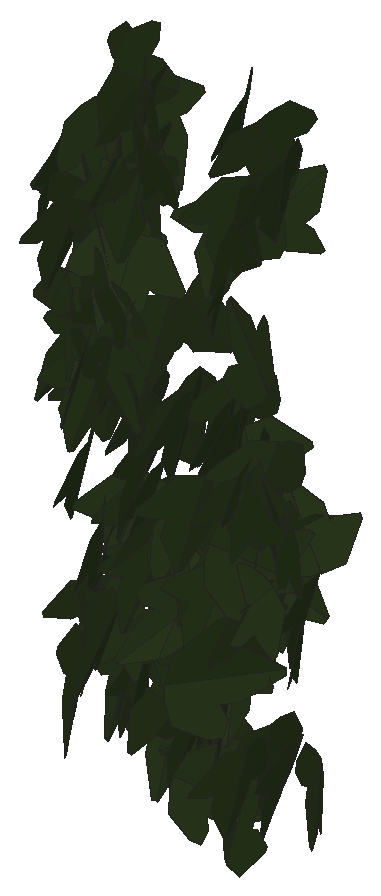
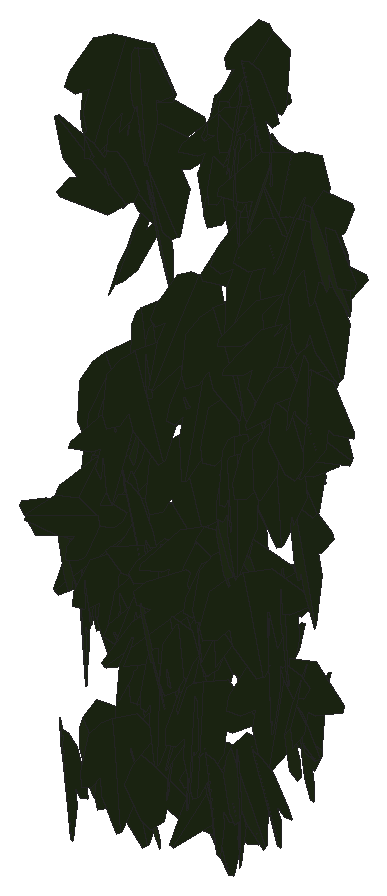
# SketchUp Ruby script. Lengths in inches.
U = 1.inch
M = Sketchup.active_model
def pt(a) = Geom::Point3d.new(a.map { |v| v * U })
def face(e, loops, mat)
  f = e.add_face(loops[0].map { |a| pt(a) })
  loops[1..].each { |l| e.add_face(l.map { |a| pt(a) }).erase! }
  f.material = f.back_material = mat if mat
  f
end
# faces: each face lists its corners as indices into pts; further lists are holes
def faces(e, pts, list, mat = nil) = list.each { |f| face(e, (f[0].is_a?(Array) ? f : [f]).map { |l| l.map { |i| pts[i] } }, mat) }
# xy, xz, yz: faces in a plane at the given z, y or x. An outline is a flat list of corners, or four numbers for a rectangle; further outlines are holes
def ring(l) = l.size == 4 ? [[l[0], l[1]], [l[2], l[1]], [l[2], l[3]], [l[0], l[3]]] : l.each_slice(2).to_a
def flat(e, list, mat, &to3) = list.each { |f| face(e, (f[0].is_a?(Array) ? f : [f]).map { |l| ring(l).map { |u, v| to3.(u, v) } }, mat) }
def xy(e, z, list, mat = nil) = flat(e, list, mat) { |x, y| [x, y, z] }
def xz(e, y, list, mat = nil) = flat(e, list, mat) { |x, z| [x, y, z] }
def yz(e, x, list, mat = nil) = flat(e, list, mat) { |y, z| [x, y, z] }
def lines(e, pts, list) = list.each { |a, b| e.add_line(pt(pts[a]), pt(pts[b])) }
# prism: a flat outline (further loops are holes) pulled along v
def prism(e, loops, v, mat = nil)
  f = face(e, loops, mat); d = Geom::Vector3d.new(v.map { |x| x * U })
  f.pushpull(f.normal.samedirection?(d) ? d.length : -d.length)
end
def box(e, o, s, mat = nil) = prism(e, [[o, [o[0] + s[0], o[1], o[2]], [o[0] + s[0], o[1] + s[1], o[2]], [o[0], o[1] + s[1], o[2]]]], [0, 0, s[2]], mat)
def at(x, y, z, deg = 0) = Geom::Transformation.translation(pt([x, y, z])) * Geom::Transformation.rotation(ORIGIN, Z_AXIS, deg.degrees)
def axes(o, x, y, z) = Geom::Transformation.new([*x, 0, *y, 0, *z, 0, *pt(o).to_a, 1])
def part(name) = M.definitions.add(name)
# library, detail: a bought-in or finely detailed component or shape, given as its bounding box
def library(name, o, s) = part(name).tap { |d| box(d.entities, o, s) }
def detail(e, o, s) = box(e.add_group.entities, o, s)
def put(e, d, t, mat = nil) = e.add_instance(d, t).tap { |i| i.material = mat if mat }
def group(e, t, mat = nil) = e.add_group.tap { |g| g.transformation = t; g.material = mat if mat }.entities
root = M.entities
M.materials.add("efeu2").color = [43, 57, 29]
c1 = part("ivyleaf_10")
p = [[0,0.5,-0.03],[-0.0625,2.02,-0.43],[-0.19,2.01,-0.46],[-0.54,1.05,-0.29],[-0.52,0.625,-0.18],[-0.83,0.76,-0.28],
  [-1.16,0.64,-0.33],[-1.15,0.33,-0.24],[-0.77,-0.39,0.02],[-0.3,-0.51,0.16],[0.04,-0.48,0.23],[-0.02,2.01,-0.4375],
  [-0.06,2.01,-0.43],[0.04,-0.49,0.23],[0.67,-0.49,0.14],[1.38,0.36,-0.2],[1.375,0.51,-0.24],[0.81,0.65,-0.19],
  [0.62,0.59,-0.15],[0.6,1.09,-0.28],[0.5,1.23,-0.31]]
faces(c1.entities,p,[[0,1,2,3,4,5,6,7,8,9,10],[11,12,0,13,14,15,16,17,18,19,20]],"efeu2")
put(root,c1,axes([506.66,136.89,179.43],[-0.21643,0.61106,0.11079],[0.02781,-0.10366,0.66875],[0.66932,0.2019,0.00804]))
put(root,c1,axes([505.3125,136.93,178.44],[0.13543,-0.68489,-0.04451],[-0.00339,0.0447,-0.69813],[0.68632,0.13537,0.00533]))
put(root,c1,axes([504.81,136.71,182.55],[-0.5524,0.19619,0.39944],[-0.38272,0.11547,-0.58598],[-0.22709,-0.67183,0.01593]))
put(root,c1,axes([504.36,137.08,181.83],[-0.27871,-0.62264,0.16039],[0.01934,-0.18285,-0.67622],[0.64267,-0.26452,0.08991]))
put(root,c1,axes([506.47,136.64,181.91],[0.09655,-0.53787,-0.44191],[0.02466,0.44851,-0.54051],[0.69569,0.05875,0.08049]))
put(root,c1,axes([503.95,136.75,179.9375],[-0.43441,0.15384,0.56092],[-0.56008,0.07816,-0.4552],[-0.15686,-0.70515,0.07191]))
put(root,c1,axes([502.98,137.33,173.17],[0.15149,-0.37032,0.60658],[0.43847,-0.43939,-0.37776],[0.5593,0.44477,0.13185]))
put(root,c1,axes([505.91,136.34,174.26],[0.04487,0.07021,0.77625],[0.10002,0.77059,-0.07548],[-0.77297,0.10379,0.03529]))
put(root,c1,axes([506.24,136.95,178.48],[0.13482,-0.67541,-0.14371],[-0.01967,0.14261,-0.68868],[0.69025,0.13599,0.00844]))
put(root,c1,axes([506.55,137.01,175.625],[0.51797,-0.07969,-0.36521],[-0.37616,0.04577,-0.50552],[0.0987,0.59265,-0.01006]))
put(root,c1,axes([503.46,137.4375,173.97],[0.14528,-0.35829,0.54775],[0.24523,-0.49042,-0.38583],[0.60685,0.28396,0.02478]))
put(root,c1,axes([504.13,137.08,180.47],[0.63313,0.2487,-0.1297],[-0.14202,0.00812,-0.67771],[-0.24187,0.64623,0.05843]))
put(root,c1,axes([503.55,137.05,178.72],[-0.56265,0.15192,-0.34681],[0.32056,-0.13943,-0.58114],[-0.20149,-0.64607,0.04387]))
put(root,c1,axes([503.22,137.18,178.59],[0.39732,-0.54573,0.04905],[0.02266,-0.04417,-0.675],[0.54746,0.3979,-0.00766]))
put(root,c1,axes([506.6,137.27,177.81],[-0.23091,-0.6062,0.20907],[0.01135,-0.22605,-0.64287],[0.64114,-0.21432,0.08668]))
put(root,c1,axes([505.92,137.08,178.4],[0.16394,-0.6525,-0.11936],[-0.00844,0.12089,-0.67245],[0.66327,0.16282,0.02095]))
put(root,c1,axes([506.42,137.01,177.4375],[-0.29178,-0.59657,-0.15254],[0.05098,0.14482,-0.66388],[0.61365,-0.29569,-0.01738]))
put(root,c1,axes([505.33,137.23,176.86],[-0.25597,-0.62666,0.1293],[-0.01982,-0.13143,-0.67622],[0.63955,-0.25488,0.03079]))
put(root,c1,axes([503.45,137.03,181.2],[-0.69675,-0.05569,0.03148],[-0.03158,-0.00006,-0.69896],[0.05563,-0.69746,-0.00245]))
put(root,c1,axes([504.34,137.17,183.06],[0.02732,-0.69814,-0.03875],[0.00552,0.039,-0.69864],[0.6992,0.02697,0.00703]))
put(root,c1,axes([506.05,137.34,181.61],[-0.46263,-0.44426,0.27239],[-0.09232,-0.2886,-0.62751],[0.51287,-0.45269,0.13274]))
put(root,c1,axes([506.11,137.22,172.65],[-0.06613,-0.65872,0.04144],[0.00583,-0.04223,-0.66195],[0.65999,-0.06563,0.01]))
put(root,c1,axes([506.07,137.29,182.04],[-0.1986,-0.65229,0.13406],[0.03584,-0.15016,-0.67754],[0.66495,-0.18672,0.07656]))
put(root,c1,axes([506.64,136.89,177.4],[0.06855,-0.55851,-0.40083],[0.15609,0.40495,-0.53754],[0.6695,-0.03722,0.16637]))
put(root,c1,axes([503.87,137.39,179],[0.10163,-0.64984,0.18183],[0.03825,-0.17804,-0.65766],[0.67371,0.10813,0.00991]))
put(root,c1,axes([504.1,137.14,182.08],[0.0796,-0.68003,-0.18076],[-0.01267,0.1805,-0.68462],[0.70353,0.08019,0.00812]))
put(root,c1,axes([503.42,137.125,181.47],[-0.35345,0.60457,-0.05381],[0.01586,-0.05305,-0.70019],[-0.60676,-0.35356,0.01305]))
put(root,c1,axes([504.27,136.8,183.66],[-0.04668,-0.43629,-0.5854],[0.18974,0.55919,-0.43189],[0.70502,-0.17938,0.07747]))
put(root,c1,axes([503.72,137.11,179.66],[-0.64262,0.23144,0.02187],[-0.02769,-0.01237,-0.6827],[-0.23081,-0.64287,0.02101]))
put(root,c1,axes([504.39,137.2,182.12],[-0.03664,-0.68496,-0.10572],[0.03027,0.10418,-0.6855],[0.6924,-0.0408,0.02437]))
put(root,c1,axes([502.67,137.4,181.62],[0.28007,-0.6353,0.11245],[0.03092,-0.10923,-0.69412],[0.64443,0.28134,-0.01556]))
put(root,c1,axes([505.82,137.27,180.87],[0.34369,-0.60969,-0.07957],[-0.01815,0.08106,-0.69948],[0.61459,0.34334,0.02384]))
put(root,c1,axes([505.13,137.5,173.1],[0.07976,-0.62324,0.17864],[0.00084,-0.17988,-0.62797],[0.64834,0.07691,-0.02116]))
put(root,c1,axes([503.51,137.34,181.25],[0.69596,-0.00157,-0.05339],[-0.05322,0.03876,-0.69489],[0.00453,0.69693,0.03853]))
put(root,c1,axes([504.35,137.33,182.99],[-0.4304,0.54258,-0.14674],[-0.00583,-0.18912,-0.68218],[-0.56204,-0.41354,0.11945]))
put(root,c1,axes([502.78,137.47,180.58],[0.01162,-0.69001,0.11879],[-0.00644,-0.11891,-0.69006],[0.70013,0.01036,-0.00832]))
put(root,c1,axes([503.91,137.43,181.92],[0.58075,-0.39263,-0.0221],[-0.02788,-0.00178,-0.70081],[0.39226,0.58117,-0.01708]))
put(root,c1,axes([506.32,137.23,177.64],[0.14089,-0.62519,-0.23745],[0.00462,0.24357,-0.63855],[0.66874,0.13003,0.05444]))
put(root,c1,axes([502.94,137.74,178.64],[-0.00213,-0.4887,0.47237],[-0.00674,-0.47234,-0.4887],[0.67965,-0.00621,-0.00337]))
put(root,c1,axes([503.21,137.59,178.09],[-0.19051,-0.60733,0.2591],[0.0341,-0.27836,-0.6274],[0.65941,-0.16107,0.10731]))
put(root,c1,axes([503.77,137.44,182.36],[-0.35837,0.49503,-0.3433],[0.20812,-0.27312,-0.61108],[-0.56532,-0.41435,-0.00735]))
put(root,c1,axes([504.45,137.52,179.38],[-0.25696,-0.62563,0.16499],[0.00234,-0.17842,-0.67292],[0.64701,-0.24782,0.06796]))
put(root,c1,axes([504.97,137.24,178.22],[-0.08665,-0.63688,-0.23448],[0.10679,0.22065,-0.63877],[0.67022,-0.1175,0.07147]))
put(root,c1,axes([504.88,137.65,174.63],[0.34102,0.2431,-0.52089],[-0.41829,-0.31049,-0.41875],[-0.39428,0.53965,-0.00628]))
put(root,c1,axes([506.3125,137.24,175.17],[-0.10941,-0.60226,-0.2658],[0.06667,0.25792,-0.61186],[0.65492,-0.12687,0.01789]))
put(root,c1,axes([505.4375,136.97,172.13],[0.06842,0.33467,0.54829],[0.08467,0.52145,-0.35406],[-0.66908,0.10021,0.01126]))
put(root,c1,axes([503.37,137.33,175.45],[0.22157,-0.58135,-0.21067],[-0.00976,0.22047,-0.61866],[0.61826,0.21182,0.06573]))
put(root,c1,axes([506.7,137.37,182.54],[0.0611,-0.67943,-0.17144],[-0.0158,0.17071,-0.68217],[0.70055,0.06311,-0.00044]))
put(root,c1,axes([504.02,137.34,183.48],[0.5103,-0.4078,-0.26684],[-0.14992,0.23627,-0.64778],[0.46371,0.52515,0.08422]))
put(root,c1,axes([505.46,137.71,173.59],[0.36769,-0.41825,0.37265],[0.27909,-0.24972,-0.55565],[0.4857,0.46011,0.03718]))
put(root,c1,axes([502.87,137.85,173.57],[0.05963,-0.17735,0.64298],[0.44796,-0.46763,-0.17053],[0.49417,0.4453,0.07699]))
put(root,c1,axes([505.51,137.66,175.19],[-0.30867,-0.51924,0.28521],[-0.10029,-0.27116,-0.6022],[0.58386,-0.32108,0.04734]))
put(root,c1,axes([506.15,136.9375,176.25],[0.00906,0.43631,0.61013],[0.01633,0.60992,-0.4364],[-0.74991,0.01856,-0.00214]))
put(root,c1,axes([506.125,137.72,175],[0.0423,0.42577,-0.44116],[-0.2339,-0.38654,-0.42429],[-0.60549,0.17906,0.13308]))
put(root,c1,axes([506.23,137.36,177.4],[-0.53939,0.42186,0.01176],[-0.00666,0.01057,-0.68476],[-0.42198,-0.53942,-0.00423]))
put(root,c1,axes([502.99,137.48,176.6],[0.21073,-0.62079,-0.12843],[-0.0454,0.12022,-0.65556],[0.6323,0.21552,-0.00427]))
put(root,c1,axes([502.98,137.7,179.27],[0.16354,0.59311,-0.30164],[-0.06851,-0.29395,-0.61515],[-0.66187,0.17698,-0.01085]))
put(root,c1,axes([504.09,137.43,182.22],[0.20776,-0.62379,-0.25004],[-0.0017,0.26123,-0.65311],[0.67204,0.1935,0.07565]))
put(root,c1,axes([504.3,137.42,177.92],[-0.57645,0.16029,0.35396],[-0.3481,0.06832,-0.59786],[-0.17264,-0.67299,0.02361]))
put(root,c1,axes([503.375,137.38,182.28],[0.32176,0.59895,0.15796],[-0.08213,0.21767,-0.6581],[-0.61396,0.28477,0.17081]))
put(root,c1,axes([504.27,137.375,182.78],[0.04732,0.67843,0.19217],[0.013,0.19173,-0.68008],[-0.705,0.04907,0.00036]))
put(root,c1,axes([505.43,137.9375,174.625],[-0.27454,-0.26666,0.55039],[-0.30057,-0.46658,-0.37599],[0.53263,-0.40075,0.07152]))
put(root,c1,axes([505.75,137.56,171.06],[0.56193,-0.36379,0.02764],[-0.01442,0.02857,0.66921],[-0.36455,-0.56188,0.01613]))
put(root,c1,axes([503.05,137.53,181.3],[-0.61607,-0.2928,-0.13396],[0.12606,0.0468,-0.68201],[0.29628,-0.62872,0.01162]))
put(root,c1,axes([506.63,137.48,176.46],[0.5599,-0.21536,-0.27537],[-0.1674,0.29128,-0.56818],[0.30689,0.55179,0.19246]))
put(root,c1,axes([506.35,137.45,183.09],[-0.32834,-0.5543,-0.27303],[0.12253,0.24464,-0.644],[0.60562,-0.35001,-0.01773]))
put(root,c1,axes([503.62,137.625,174.07],[0.49835,-0.14972,-0.43723],[-0.4207,0.11922,-0.52033],[0.19131,0.65216,-0.00526]))
put(root,c1,axes([505.55,137.72,174],[0.64382,-0.05207,0.10376],[0.10279,-0.01602,-0.64588],[0.05395,0.65193,-0.00759]))
put(root,c1,axes([503.875,137.91,176.83],[0.20724,-0.64225,0.25846],[0.07814,-0.24636,-0.67486],[0.68788,0.22147,-0.00121]))
put(root,c1,axes([504.67,137.83,174.42],[-0.2093,-0.60601,0.18091],[0.02161,-0.1973,-0.63591],[0.63206,-0.19393,0.08164]))
put(root,c1,axes([505.6875,137.78,178.36],[-0.24386,-0.62024,0.12857],[-0.0201,-0.13012,-0.66585],[0.63311,-0.24303,0.02838]))
put(root,c1,axes([504.05,137.8,176.4],[0.21898,-0.62826,0.04849],[0.00191,-0.05068,-0.66517],[0.63013,0.21848,-0.01484]))
put(root,c1,axes([502.77,137.7,179.05],[-0.67491,-0.02529,-0.01054],[0.01505,-0.1251,-0.66361],[0.02289,-0.66329,0.12556]))
put(root,c1,axes([505.3,137.59,173.5],[0.33173,-0.53622,-0.23848],[-0.04541,0.24967,-0.62455],[0.5851,0.32339,0.08674]))
put(root,c1,axes([503.99,137.91,175.06],[-0.14234,-0.59627,0.23499],[-0.02784,-0.23473,-0.61249],[0.6403,-0.14276,0.02561]))
put(root,c1,axes([504.43,137.79,175.77],[-0.34638,0.01985,0.57524],[-0.54168,-0.23825,-0.31795],[0.19462,-0.62778,0.13886]))
put(root,c1,axes([503.14,137.61,179.3],[-0.6013,0.30957,-0.03744],[0.02574,-0.03178,-0.67611],[-0.31076,-0.60162,0.01645]))
put(root,c1,axes([503.3,137.625,180.1875],[0.18959,0.66435,0.01771],[-0.00909,0.021,-0.69073],[-0.66453,0.18926,0.0145]))
put(root,c1,axes([505.69,137.6875,175.93],[-0.64774,-0.10658,0.07529],[-0.06974,-0.0496,-0.63234],[0.12041,-0.60207,0.03876]))
put(root,c1,axes([505.07,137.62,174.07],[0.11277,-0.61552,-0.23177],[-0.06724,0.22313,-0.62529],[0.65426,0.12902,-0.02431]))
put(root,c1,axes([504.75,137.61,175.9],[0.18241,0.63323,0.07754],[0.02202,0.07435,-0.65898],[-0.63758,0.18374,-0.00057]))
put(root,c1,axes([503.67,137.54,181.11],[-0.27429,-0.55238,-0.32377],[0.12825,0.29768,-0.61654],[0.6273,-0.30239,-0.01551]))
put(root,c1,axes([503.24,137.77,177.93],[-0.27374,-0.60983,-0.01375],[0.00418,0.0132,-0.66845],[0.60997,-0.27377,-0.00159]))
put(root,c1,axes([504.98,137.52,179.74],[-0.10272,-0.55324,-0.38747],[0.16497,0.3595,-0.55705],[0.65498,-0.17731,0.07954]))
put(root,c1,axes([503.23,137.68,179.77],[0.11996,0.67336,0.03139],[0.01423,0.02935,-0.68391],[-0.67394,0.12048,-0.00885]))
put(root,c1,axes([505.81,137.87,172.09],[-0.18802,-0.62016,0.0716],[-0.0099,-0.0718,-0.64794],[0.6242,-0.18794,0.01129]))
put(root,c1,axes([505.74,137.68,183.25],[0.12879,-0.54481,-0.2731],[-0.07275,0.25402,-0.57991],[0.64911,0.13657,-0.01081]))
put(root,c1,axes([503.15,137.74,174.23],[-0.46303,-0.45718,-0.09759],[0.06183,0.07626,-0.65061],[0.46337,-0.46702,-0.01071]))
put(root,c1,axes([505.58,137.7,174.56],[0.27113,-0.54341,-0.23966],[-0.00797,0.2601,-0.59877],[0.59385,0.25159,0.10138]))
put(root,c1,axes([505.75,137.84,175.02],[-0.59626,-0.15913,0.3482],[-0.33562,-0.09279,-0.61713],[0.18419,-0.68422,0.00271]))
put(root,c1,axes([506.79,137.97,175.43],[0.2093,-0.63045,0.02736],[0.00537,-0.02704,-0.66427],[0.63102,0.20934,-0.00342]))
put(root,c1,axes([505.78,137.86,176.3],[0.49233,-0.41894,-0.11947],[-0.04626,0.129,-0.64295],[0.43318,0.48992,0.06713]))
put(root,c1,axes([505.875,137.74,177.52],[0.21091,0.64012,0.1146],[0.00102,0.12015,-0.673],[-0.6503,0.2078,0.03612]))
put(root,c1,axes([506.29,138.1,172.38],[0.19805,-0.60292,0.15583],[0.03265,-0.15325,-0.6344],[0.62188,0.20006,-0.01633]))
put(root,c1,axes([503.84,138.03,175.91],[-0.23651,-0.61153,0.09292],[0.01605,-0.10552,-0.65356],[0.61834,-0.23116,0.0525]))
put(root,c1,axes([505.91,137.91,175.06],[-0.46089,-0.42098,-0.05067],[0.04782,0.02447,-0.62327],[0.45519,-0.42882,0.01417]))
put(root,c1,axes([505.17,137.66,175.34],[-0.16602,-0.43543,-0.47158],[0.24756,0.40598,-0.46201],[0.5922,-0.29178,0.06092]))
put(root,c1,axes([505.39,138.3,174.4],[-0.05738,0.38291,-0.5213],[0.00986,-0.52277,-0.38507],[-0.64675,-0.04194,0.04038]))
put(root,c1,axes([503.8,137.94,177.68],[0.10256,-0.63779,-0.1852],[0.00128,0.18759,-0.6453],[0.66414,0.09813,0.02984]))
put(root,c1,axes([505.94,137.67,175.7],[0.33396,0.29565,0.55088],[0.30073,0.47159,-0.4354],[-0.54812,0.43887,0.09675]))
put(root,c1,axes([504.08,137.89,175.59],[-0.18306,-0.58618,-0.2297],[0.06546,0.22019,-0.61409],[0.62617,-0.19439,-0.00295]))
put(root,c1,axes([505.12,137.76,175.27],[0.37249,0.3458,0.47277],[0.30161,0.36705,-0.50611],[-0.50212,0.47701,0.04671]))
put(root,c1,axes([504.97,137.85,173.24],[0.30507,-0.48239,-0.29893],[-0.00373,0.33767,-0.54871],[0.56749,0.26154,0.15709]))
put(root,c1,axes([503.45,138.18,175.71],[-0.4348,-0.47216,0.13175],[0.01669,-0.19027,-0.62679],[0.48991,-0.41256,0.13828]))
put(root,c1,axes([503.19,138.15,172.98],[0.54098,-0.36291,0.04755],[0.04815,-0.01356,-0.65125],[0.36283,0.5429,0.01552]))
put(root,c1,axes([506.07,138.01,181.38],[0.48426,-0.01654,-0.40869],[0.42289,-0.03737,0.4663],[-0.04002,-0.59504,-0.01793]))
put(root,c1,axes([505.08,138.12,174.5],[-0.61984,-0.09076,-0.18297],[0.19865,-0.13209,-0.60746],[0.04745,-0.63264,0.15308]))
put(root,c1,axes([503.7,138.02,177.46],[0.03296,-0.63429,-0.20279],[-0.00242,0.20292,-0.6351],[0.66591,0.03213,0.00773]))
put(root,c1,axes([505.24,138.15,174.75],[0.26777,-0.58215,-0.12562],[-0.05567,0.11266,-0.64077],[0.59294,0.27347,-0.00343]))
put(root,c1,axes([503.45,138.31,172.96],[0.14258,-0.62096,0.10312],[0.01109,-0.10324,-0.637],[0.62936,0.1425,-0.01214]))
put(root,c1,axes([503.95,138.25,172.23],[0.63115,-0.14606,0.04699],[0.04708,-0.00498,-0.6478],[0.14603,0.63288,0.00574]))
put(root,c1,axes([504.76,137.83,174.93],[-0.26002,-0.289,-0.60205],[0.44575,0.406,-0.3874],[0.49729,-0.51502,0.03244]))
put(root,c1,axes([506.5,138.07,174.7],[0.34716,-0.50532,-0.24475],[-0.04641,0.26095,-0.60459],[0.55955,0.33516,0.1017]))
put(root,c1,axes([505.81,138.21,172.51],[-0.14859,-0.62434,-0.05258],[0.00864,0.05199,-0.64177],[0.62649,-0.1488,-0.00362]))
put(root,c1,axes([503.05,138.09,175.14],[0.2576,-0.5364,-0.28712],[-0.0547,0.29012,-0.59107],[0.60595,0.25422,0.06871]))
put(root,c1,axes([504.93,138.38,172.4],[-0.32827,-0.09847,0.53734],[-0.47668,-0.25459,-0.33787],[0.26685,-0.57592,0.05748]))
put(root,c1,axes([506.27,137.86,175.91],[-0.00779,-0.16656,0.60983],[0.13535,0.57349,0.17102],[-0.64428,0.12249,0.02855]))
put(root,c1,axes([503.98,138.01,172.64],[-0.14347,-0.46592,-0.42649],[0.24891,0.36026,-0.4773],[0.58053,-0.26961,0.09925]))
put(root,c1,axes([506.6,138.27,175.85],[0.38509,0.43899,0.14838],[-0.097,-0.11086,0.58818],[0.489,-0.3677,-0.00018]))
put(root,c1,axes([506.63,138.28,172.13],[0.49527,-0.41563,-0.07974],[0.02864,0.15539,-0.63201],[0.42224,0.47697,0.13641]))
put(root,c1,axes([504.42,138.09,173.95],[0.14432,-0.5281,-0.3445],[0.11954,0.36991,-0.51698],[0.61909,0.05168,0.18013]))
put(root,c1,axes([504.12,138.32,173.75],[-0.16604,-0.61112,-0.13191],[0.04569,0.12426,-0.63318],[0.62352,-0.17185,0.01127]))
put(root,c1,axes([504.9,138.28,174.02],[0.04464,-0.60653,-0.22663],[0.00159,0.22727,-0.60793],[0.64749,0.04126,0.01711]))
put(root,c1,axes([503.43,138.33,172.89],[0.29891,-0.53353,-0.20138],[-0.00132,0.22672,-0.60262],[0.57026,0.28018,0.10416]))
put(root,c1,axes([503.82,138.49,172.83],[0.51866,-0.36951,0.01274],[0.07055,0.07736,-0.62829],[0.36294,0.51302,0.10392]))
put(root,c1,axes([504.29,138.33,173.53],[0.33917,-0.46322,-0.29349],[-0.02949,0.32918,-0.55364],[0.54758,0.30465,0.15197]))
